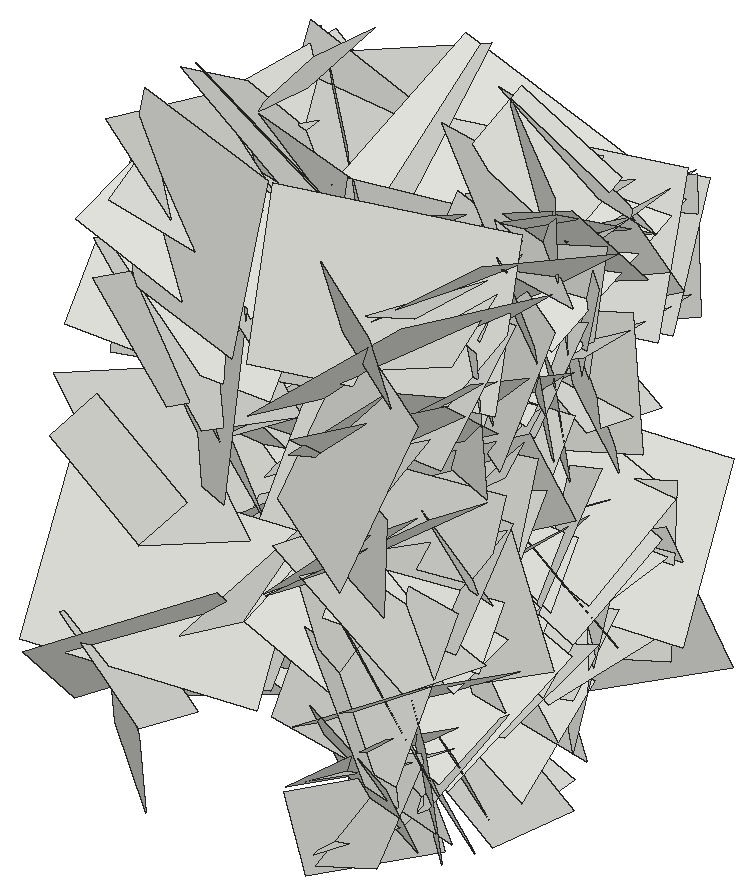
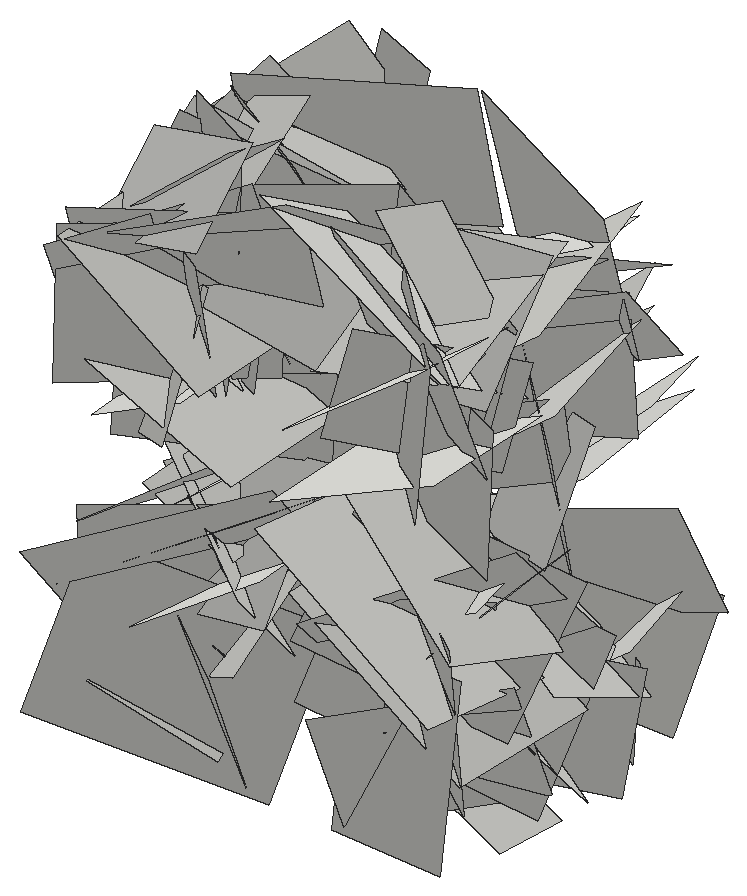
# SketchUp Ruby script. Lengths in inches.
U = 1.inch
M = Sketchup.active_model
def pt(a) = Geom::Point3d.new(a.map { |v| v * U })
def face(e, loops, mat)
  f = e.add_face(loops[0].map { |a| pt(a) })
  loops[1..].each { |l| e.add_face(l.map { |a| pt(a) }).erase! }
  f.material = f.back_material = mat if mat
  f
end
# faces: each face lists its corners as indices into pts; further lists are holes
def faces(e, pts, list, mat = nil) = list.each { |f| face(e, (f[0].is_a?(Array) ? f : [f]).map { |l| l.map { |i| pts[i] } }, mat) }
# xy, xz, yz: faces in a plane at the given z, y or x. An outline is a flat list of corners, or four numbers for a rectangle; further outlines are holes
def ring(l) = l.size == 4 ? [[l[0], l[1]], [l[2], l[1]], [l[2], l[3]], [l[0], l[3]]] : l.each_slice(2).to_a
def flat(e, list, mat, &to3) = list.each { |f| face(e, (f[0].is_a?(Array) ? f : [f]).map { |l| ring(l).map { |u, v| to3.(u, v) } }, mat) }
def xy(e, z, list, mat = nil) = flat(e, list, mat) { |x, y| [x, y, z] }
def xz(e, y, list, mat = nil) = flat(e, list, mat) { |x, z| [x, y, z] }
def yz(e, x, list, mat = nil) = flat(e, list, mat) { |y, z| [x, y, z] }
def lines(e, pts, list) = list.each { |a, b| e.add_line(pt(pts[a]), pt(pts[b])) }
# prism: a flat outline (further loops are holes) pulled along v
def prism(e, loops, v, mat = nil)
  f = face(e, loops, mat); d = Geom::Vector3d.new(v.map { |x| x * U })
  f.pushpull(f.normal.samedirection?(d) ? d.length : -d.length)
end
def box(e, o, s, mat = nil) = prism(e, [[o, [o[0] + s[0], o[1], o[2]], [o[0] + s[0], o[1] + s[1], o[2]], [o[0], o[1] + s[1], o[2]]]], [0, 0, s[2]], mat)
def at(x, y, z, deg = 0) = Geom::Transformation.translation(pt([x, y, z])) * Geom::Transformation.rotation(ORIGIN, Z_AXIS, deg.degrees)
def axes(o, x, y, z) = Geom::Transformation.new([*x, 0, *y, 0, *z, 0, *pt(o).to_a, 1])
def part(name) = M.definitions.add(name)
# library, detail: a bought-in or finely detailed component or shape, given as its bounding box
def library(name, o, s) = part(name).tap { |d| box(d.entities, o, s) }
def detail(e, o, s) = box(e.add_group.entities, o, s)
def put(e, d, t, mat = nil) = e.add_instance(d, t).tap { |i| i.material = mat if mat }
def group(e, t, mat = nil) = e.add_group.tap { |g| g.transformation = t; g.material = mat if mat }.entities
root = M.entities
c1 = part("Component\#6")
p = [[0.01,0,0],[0,3.24,4.54],[4.32,3.24,4.54],[4.33,0,0]]
faces(c1.entities,p,[[0,1,2,3]])
put(root,c1,axes([14.53,182.77,28.15],[-0.11013,-1.0722,-0.31704],[-0.03816,-0.31503,1.07721],[1.18456,-0.10983,0.00522]))
put(root,c1,axes([14.53,176.05,33.17],[0.01986,0.50916,-0.88553],[-0.06176,-0.8837,-0.50934],[1.08099,-0.05984,-0.01283]))
put(root,c1,axes([18.5,182.27,37.76],[0.22679,0.05489,-0.89691],[0.06736,-0.9206,-0.04118],[-0.95012,-0.05216,-0.217]))
put(root,c1,axes([14.53,174.9,23.69],[-0.06803,0.90477,0.33383],[0.16872,0.33992,-0.89067],[1.00823,0.00417,0.17157]))
put(root,c1,axes([18.5,173.11,21.9],[0.05319,-0.68826,0.19248],[0.04456,0.19546,0.68797],[-0.75624,-0.03689,0.05408]))
put(root,c1,axes([18.5,178.15,33.23],[-0.08938,-0.00525,-0.60269],[0.06829,-0.60515,-0.00374],[-0.63521,-0.06432,0.0844]))
put(root,c1,axes([18.5,176.44,21.6],[0.04345,0.60879,-0.00304],[-0.10651,0.00376,-0.60183],[-0.63647,0.04093,0.10051]))
put(root,c1,axes([14.53,183.67,38.38],[0.04708,0.10578,-1.15378],[-0.2342,-1.13267,-0.11235],[1.2056,-0.22416,0.02323]))
put(root,c1,axes([14.53,173.31,35.98],[-0.01252,1.07454,-0.37217],[-0.12805,-0.37127,-1.06811],[1.19858,-0.02844,-0.11799]))
put(root,c1,axes([14.53,174.78,20.26],[0.10048,-0.39109,0.79293],[0.10042,0.79738,0.38196],[0.93179,-0.04376,-0.12667]))
put(root,c1,axes([18.5,180.68,27.18],[0.06604,-0.60003,0.10008],[-0.10227,0.08959,0.59716],[-0.63666,-0.07663,-0.08554]))
put(root,c1,axes([18.5,170.73,19.61],[0.06378,-0.15247,0.68566],[0.07422,0.68605,0.14641],[-0.74085,0.05561,0.0737]))
put(root,c1,axes([14.53,178.01,21.81],[0.00864,0.40014,0.99077],[-0.02339,0.99065,-0.39991],[1.13239,0.01741,-0.01582]))
put(root,c1,axes([18.5,178.13,40.15],[0.04908,0.64392,0.19174],[0.08573,0.18545,-0.64234],[-0.70699,0.06719,-0.06458]))
put(root,c1,axes([14.53,171.95,33.74],[-0.07102,0.70639,0.8167],[0.11892,0.8184,-0.69866],[1.13841,-0.04142,0.12393]))
put(root,c1,axes([18.5,176.07,37.03],[0.15674,-0.62528,-0.09698],[-0.10666,-0.12156,0.63036],[-0.66219,-0.12843,-0.12449]))
put(root,c1,axes([18.5,180.42,25.12],[0.17902,-0.88337,-0.09354],[0.21931,-0.05348,0.8786],[-0.91571,-0.1855,0.19214]))
put(root,c1,axes([14.53,172.46,21.25],[0.14489,-0.73421,0.72244],[-0.08794,0.71856,0.74596],[1.0883,0.15581,-0.0359]))
put(root,c1,axes([14.53,171.47,32.36],[0.16942,0.96147,-0.31887],[-0.08969,-0.30901,-0.97416],[1.06999,-0.17814,-0.03117]))
put(root,c1,axes([14.53,179.35,38.14],[0.07028,1.07405,0.02302],[-0.04111,0.02544,-1.07534],[1.13802,-0.06541,-0.04027]))
put(root,c1,axes([18.5,181.39,28.46],[0.11732,-0.15238,-0.58962],[-0.01785,-0.59981,0.15186],[-0.64528,-0.01111,-0.1114]))
put(root,c1,axes([18.5,173.74,31.89],[0.15856,-0.67469,0.29232],[0.1064,0.31425,0.67394],[-0.77211,-0.09525,0.1529]))
put(root,c1,axes([14.53,173.84,39.64],[-0.13369,1.27699,-0.41872],[-0.11509,-0.42887,-1.27523],[1.41986,0.08547,-0.14279]))
put(root,c1,axes([18.5,172.58,29],[0.14706,-0.68518,0.03236],[0.10474,0.05263,0.69082],[-0.71951,-0.13238,0.10718]))
put(root,c1,axes([14.53,180.75,35.09],[-0.01445,0.08276,-1.11066],[0.1396,-1.10283,-0.0838],[1.17228,0.13235,-0.00371]))
put(root,c1,axes([14.53,182.25,27.43],[-0.1955,0.46825,-1.21407],[0.10064,-1.21809,-0.48422],[1.37564,0.15566,-0.13711]))
put(root,c1,axes([14.53,175.96,26.52],[0.03553,0.82214,0.9074],[-0.07429,0.90754,-0.81968],[1.2958,0.02948,-0.07187]))
put(root,c1,axes([14.53,172.47,36.95],[0.1233,0.89549,0.4145],[0.21728,0.38634,-0.89217],[1.02316,-0.18996,0.13951]))
put(root,c1,axes([14.53,183.25,38.77],[-0.07927,-0.40868,-1.12281],[0.1988,-1.11508,0.39337],[1.25087,0.15132,-0.13368]))
put(root,c1,axes([14.53,179.04,23.77],[0.11323,-0.75693,-0.7774],[0.09292,-0.77258,0.76428],[1.14637,0.13739,0.01483]))
put(root,c1,axes([14.53,182.77,28.7],[-0.0358,-0.11408,-1.31406],[-0.04325,-1.31377,0.1151],[1.39747,-0.04358,-0.0301]))
put(root,c1,axes([14.53,180.07,24.39],[-0.06666,-0.76105,0.92501],[0.21989,0.90537,0.75899],[1.25053,-0.19976,-0.08415]))
put(root,c1,axes([14.53,177.97,39.67],[-0.02985,0.75948,-0.84861],[0.27983,-0.8214,-0.74388],[1.17429,0.21504,0.15569]))
put(root,c1,axes([14.53,174.06,31.875],[0.08593,-0.00736,1.08266],[0.18405,1.07173,-0.00571],[1.1328,-0.17357,-0.0812]))
put(root,c1,axes([14.53,182.31,23.94],[-0.04872,-1.30982,0.04089],[0.01644,0.04037,1.31055],[1.38898,-0.04642,-0.01408]))
put(root,c1,axes([14.53,178.49,34.59],[0.00763,1.14917,-0.03145],[0.21412,-0.03223,-1.13128],[1.19962,-0.00155,0.20212]))
put(root,c1,axes([14.53,178.09,32.9],[0.18757,-0.47698,-1.21124],[-0.23196,-1.21588,0.44684],[1.36024,-0.14157,0.24323]))
put(root,c1,axes([14.53,178.68,21.25],[0.14964,-1.02559,0.91665],[-0.24358,0.89093,1.03221],[1.43757,0.25771,0.07948]))
put(root,c1,axes([14.53,169.91,24.28],[-0.0494,0.58776,1.07494],[0.25393,1.05932,-0.56884],[1.27358,-0.18841,0.15511]))
put(root,c1,axes([14.53,175.66,39.88],[-0.03914,-0.32872,-1.22009],[0.25418,-1.20026,0.31612],[1.31508,0.2222,-0.09741]))
put(root,c1,axes([14.53,177.96,25.04],[0.10915,-1.1796,-0.55067],[0.03689,-0.5497,1.18402],[1.37942,0.10803,0.01191]))
put(root,c1,axes([14.53,183.77,26.5],[0.0762,-1.33255,-0.21023],[0.04546,-0.20817,1.33413],[1.42926,0.07766,-0.03122]))
put(root,c1,axes([14.53,177.28,39.83],[0.04784,1.11638,-0.64936],[0.22797,-0.64718,-1.09769],[1.34988,0.06974,0.20839]))
put(root,c1,axes([14.53,179.625,37.91],[0.28026,0.12179,-1.29213],[0.26115,-1.29941,-0.07206],[1.35072,0.22596,0.28204]))
put(root,c1,axes([14.53,183.19,37.72],[0.19709,-1.17807,-0.70591],[0.26547,-0.67132,1.18631],[1.43137,0.28672,-0.12282]))
put(root,c1,axes([28.31,183.19,37.72],[-0.19709,-1.17807,-0.70591],[-0.26547,-0.67132,1.18631],[-1.43137,0.28672,-0.12282]))
put(root,c1,axes([28.31,179.625,37.91],[-0.28026,0.12179,-1.29213],[-0.26115,-1.29941,-0.07206],[-1.35072,0.22596,0.28204]))
put(root,c1,axes([28.31,177.28,39.83],[-0.04784,1.11638,-0.64936],[-0.22797,-0.64718,-1.09769],[-1.34988,0.06974,0.20839]))
put(root,c1,axes([28.31,183.77,26.5],[-0.0762,-1.33255,-0.21023],[-0.04546,-0.20817,1.33413],[-1.42926,0.07766,-0.03122]))
put(root,c1,axes([28.31,177.96,25.04],[-0.10915,-1.1796,-0.55067],[-0.03689,-0.5497,1.18402],[-1.37942,0.10803,0.01191]))
put(root,c1,axes([28.31,175.66,39.88],[0.03914,-0.32872,-1.22009],[-0.25418,-1.20026,0.31612],[-1.31508,0.2222,-0.09741]))
put(root,c1,axes([28.31,169.91,24.28],[0.0494,0.58776,1.07494],[-0.25393,1.05932,-0.56884],[-1.27358,-0.18841,0.15511]))
put(root,c1,axes([28.31,178.68,21.25],[-0.14964,-1.02559,0.91665],[0.24358,0.89093,1.03221],[-1.43757,0.25771,0.07948]))
put(root,c1,axes([28.31,178.09,32.9],[-0.18757,-0.47698,-1.21124],[0.23196,-1.21588,0.44684],[-1.36024,-0.14157,0.24323]))
put(root,c1,axes([28.31,178.49,34.59],[-0.00763,1.14917,-0.03145],[-0.21412,-0.03223,-1.13128],[-1.19962,-0.00155,0.20212]))
put(root,c1,axes([28.31,182.31,23.94],[0.04872,-1.30982,0.04089],[-0.01644,0.04037,1.31055],[-1.38898,-0.04642,-0.01408]))
put(root,c1,axes([28.31,174.06,31.875],[-0.08593,-0.00736,1.08266],[-0.18405,1.07173,-0.00571],[-1.1328,-0.17357,-0.0812]))
put(root,c1,axes([28.31,177.97,39.67],[0.02985,0.75948,-0.84861],[-0.27983,-0.8214,-0.74388],[-1.17429,0.21504,0.15569]))
put(root,c1,axes([28.31,180.07,24.39],[0.06666,-0.76105,0.92501],[-0.21989,0.90537,0.75899],[-1.25053,-0.19976,-0.08415]))
put(root,c1,axes([28.31,182.77,28.7],[0.0358,-0.11408,-1.31406],[0.04325,-1.31377,0.1151],[-1.39747,-0.04358,-0.0301]))
put(root,c1,axes([28.31,179.04,23.77],[-0.11323,-0.75693,-0.7774],[-0.09292,-0.77258,0.76428],[-1.14637,0.13739,0.01483]))
put(root,c1,axes([28.31,183.25,38.77],[0.07927,-0.40868,-1.12281],[-0.1988,-1.11508,0.39337],[-1.25087,0.15132,-0.13368]))
put(root,c1,axes([28.31,172.47,36.95],[-0.1233,0.89549,0.4145],[-0.21728,0.38634,-0.89217],[-1.02316,-0.18996,0.13951]))
put(root,c1,axes([28.31,175.96,26.52],[-0.03553,0.82214,0.9074],[0.07429,0.90754,-0.81968],[-1.2958,0.02948,-0.07187]))
put(root,c1,axes([28.31,182.25,27.43],[0.1955,0.46825,-1.21407],[-0.10064,-1.21809,-0.48422],[-1.37564,0.15566,-0.13711]))
put(root,c1,axes([28.31,180.75,35.09],[0.01445,0.08276,-1.11066],[-0.1396,-1.10283,-0.0838],[-1.17228,0.13235,-0.00371]))
put(root,c1,axes([24.34,172.58,29],[-0.14706,-0.68518,0.03236],[-0.10474,0.05263,0.69082],[0.71951,-0.13238,0.10718]))
put(root,c1,axes([28.31,173.84,39.64],[0.13369,1.27699,-0.41872],[0.11509,-0.42887,-1.27523],[-1.41986,0.08547,-0.14279]))
put(root,c1,axes([24.34,173.74,31.89],[-0.15856,-0.67469,0.29232],[-0.1064,0.31425,0.67394],[0.77211,-0.09525,0.1529]))
put(root,c1,axes([24.34,181.39,28.46],[-0.11732,-0.15238,-0.58962],[0.01785,-0.59981,0.15186],[0.64528,-0.01111,-0.1114]))
put(root,c1,axes([28.31,179.35,38.14],[-0.07028,1.07405,0.02302],[0.04111,0.02544,-1.07534],[-1.13802,-0.06541,-0.04027]))
put(root,c1,axes([28.31,171.47,32.36],[-0.16942,0.96147,-0.31887],[0.08969,-0.30901,-0.97416],[-1.06999,-0.17814,-0.03117]))
put(root,c1,axes([28.31,172.46,21.25],[-0.14489,-0.73421,0.72244],[0.08794,0.71856,0.74596],[-1.0883,0.15581,-0.0359]))
put(root,c1,axes([24.34,180.42,25.12],[-0.17902,-0.88337,-0.09354],[-0.21931,-0.05348,0.8786],[0.91571,-0.1855,0.19214]))
put(root,c1,axes([24.34,176.07,37.03],[-0.15674,-0.62528,-0.09698],[0.10666,-0.12156,0.63036],[0.66219,-0.12843,-0.12449]))
put(root,c1,axes([28.31,171.95,33.74],[0.07102,0.70639,0.8167],[-0.11892,0.8184,-0.69866],[-1.13841,-0.04142,0.12393]))
put(root,c1,axes([24.34,178.13,40.15],[-0.04908,0.64392,0.19174],[-0.08573,0.18545,-0.64234],[0.70699,0.06719,-0.06458]))
put(root,c1,axes([28.31,178.01,21.81],[-0.00864,0.40014,0.99077],[0.02339,0.99065,-0.39991],[-1.13239,0.01741,-0.01582]))
put(root,c1,axes([24.34,170.73,19.61],[-0.06378,-0.15247,0.68566],[-0.07422,0.68605,0.14641],[0.74085,0.05561,0.0737]))
put(root,c1,axes([24.34,180.68,27.18],[-0.06604,-0.60003,0.10008],[0.10227,0.08959,0.59716],[0.63666,-0.07663,-0.08554]))
put(root,c1,axes([28.31,174.78,20.26],[-0.10048,-0.39109,0.79293],[-0.10042,0.79738,0.38196],[-0.93179,-0.04376,-0.12667]))
put(root,c1,axes([28.31,173.31,35.98],[0.01252,1.07454,-0.37217],[0.12805,-0.37127,-1.06811],[-1.19858,-0.02844,-0.11799]))
put(root,c1,axes([28.31,183.67,38.38],[-0.04708,0.10578,-1.15378],[0.2342,-1.13267,-0.11235],[-1.2056,-0.22416,0.02323]))
put(root,c1,axes([24.34,176.44,21.6],[-0.04345,0.60879,-0.00304],[0.10651,0.00376,-0.60183],[0.63647,0.04093,0.10051]))
put(root,c1,axes([24.34,178.15,33.23],[0.08938,-0.00525,-0.60269],[-0.06829,-0.60515,-0.00374],[0.63521,-0.06432,0.0844]))
put(root,c1,axes([24.34,173.11,21.9],[-0.05319,-0.68826,0.19248],[-0.04456,0.19546,0.68797],[0.75624,-0.03689,0.05408]))
put(root,c1,axes([28.31,174.9,23.69],[0.06803,0.90477,0.33383],[-0.16872,0.33992,-0.89067],[-1.00823,0.00417,0.17157]))
put(root,c1,axes([24.34,182.27,37.76],[-0.22679,0.05489,-0.89691],[-0.06736,-0.9206,-0.04118],[0.95012,-0.05216,-0.217]))
put(root,c1,axes([28.31,176.05,33.17],[-0.01986,0.50916,-0.88553],[0.06176,-0.8837,-0.50934],[-1.08099,-0.05984,-0.01283]))
put(root,c1,axes([28.31,182.77,28.15],[0.11013,-1.0722,-0.31704],[0.03816,-0.31503,1.07721],[-1.18456,-0.10983,0.00522]))
put(root,c1,axes([28.31,185.38,28.27],[0.28552,-0.8956,-0.93898],[0.07116,-0.9481,0.92355],[-1.37362,-0.23528,-0.14733]))
put(root,c1,axes([24.34,175.43,34.87],[-0.0411,0.62613,0.35799],[-0.03637,0.3565,-0.62724],[0.76365,0.05068,-0.01061]))
put(root,c1,axes([24.34,173.67,32.24],[-0.05341,-0.65994,-0.37026],[-0.06447,-0.36634,0.66124],[0.79951,-0.07362,0.02859]))
put(root,c1,axes([28.31,174.01,26.46],[0.07872,-0.97306,0.24072],[-0.0738,0.23579,0.97461],[-1.05998,-0.08868,-0.04998]))
put(root,c1,axes([28.31,170.16,39.2],[0.24703,1.2789,-0.21613],[0.13589,-0.24123,-1.28918],[-1.36812,0.20696,-0.16707]))
put(root,c1,axes([24.34,173.15,22.23],[0.01199,-0.5915,0.12784],[0.10227,0.12799,0.58366],[0.63327,-0.00947,-0.09668]))
put(root,c1,axes([28.31,167.34,31.77],[0.2501,0.51374,1.1242],[0.05799,1.13903,-0.532],[-1.3089,0.14863,0.19123]))
put(root,c1,axes([24.34,174.375,32.02],[-0.18574,0.64681,-0.5499],[-0.00393,-0.56207,-0.65994],[0.8999,0.13105,-0.11638]))
put(root,c1,axes([24.34,171.42,39.46],[0.01769,0.21401,-0.61924],[0.03571,-0.6189,-0.21298],[0.69357,0.02641,0.02676]))
put(root,c1,axes([24.34,180.11,41],[-0.0874,0.13713,-0.78202],[-0.02965,-0.78624,-0.13492],[0.84107,-0.01347,-0.08602]))
put(root,c1,axes([28.31,182.1,27.04],[0.18817,-1.1788,-0.21223],[0.10509,-0.19936,1.19019],[-1.26526,-0.19187,0.06729]))
put(root,c1,axes([28.31,177.13,31.79],[0.078,-0.30439,1.03044],[0.07955,1.03178,0.29943],[-1.13614,0.05135,0.09171]))
put(root,c1,axes([28.31,172.13,35.78],[-0.07615,0.65901,-0.5201],[-0.04859,-0.52431,-0.658],[-0.88857,-0.02781,0.08055]))
put(root,c1,axes([28.31,172.625,27.43],[0.01975,0.58315,0.74345],[-0.01761,0.74368,-0.58292],[-1.00141,-0.00157,0.02491]))
put(root,c1,axes([28.31,173.5,20.5],[0.29119,-0.77592,0.90535],[-0.00734,0.92801,0.79744],[-1.26387,-0.18415,0.20396]))
put(root,c1,axes([28.31,181.8125,37.17],[0.0246,-0.63961,0.56311],[-0.17949,0.54862,0.63013],[-0.88529,-0.129,-0.11211]))
put(root,c1,axes([24.34,177.7,39.03],[-0.08239,-0.33737,-0.64844],[0.10668,-0.65083,0.32654],[0.76743,0.05425,-0.11501]))
put(root,c1,axes([28.31,176.41,32.2],[-0.11408,-0.0942,-0.79779],[-0.0272,-0.8041,0.09841],[-0.85109,0.03832,0.10379]))
put(root,c1,axes([28.31,171.36,22.89],[-0.02535,0.88672,0.32576],[0.06435,0.32663,-0.88464],[-0.99927,-0.00146,-0.06523]))
put(root,c1,axes([28.31,178.05,19.9375],[0.14578,-1.0409,0.22357],[0.02192,0.228,1.04879],[-1.1283,-0.13006,0.04926]))
put(root,c1,axes([28.31,180.04,24.28],[-0.15161,0.71603,-0.23582],[-0.04269,-0.24694,-0.72538],[-0.79796,-0.12284,0.08362]))
put(root,c1,axes([24.34,173.29,20.87],[0.09428,-0.62013,-0.08152],[0.03551,-0.0775,0.6261],[0.66205,0.09247,-0.02197]))
put(root,c1,axes([24.34,173.36,27.66],[-0.12062,0.63946,0.63128],[-0.06443,0.62939,-0.6485],[0.9503,0.12384,0.03616]))
put(root,c1,axes([28.31,175.14,30.45],[0.22771,0.17317,-1.07869],[-0.0194,-1.09862,-0.18001],[-1.15789,0.05246,-0.20912]))
put(root,c1,axes([28.31,184.3,37.98],[0.01849,-0.42221,-1.00939],[0.24573,-0.98518,0.41609],[-1.13346,-0.22047,0.07374]))
put(root,c1,axes([24.34,172.01,32.68],[0.01531,-0.04852,-0.71126],[0.05574,-0.70939,0.04946],[0.75363,0.05345,0.01079]))
put(root,c1,axes([28.31,172,20.82],[0.19013,-0.4174,1.11707],[0.18593,1.12659,0.39279],[-1.25031,0.10406,0.22828]))
put(root,c1,axes([28.31,178.01,36.42],[-0.04909,-0.68925,0.58112],[0.09024,0.57594,0.68989],[-0.95135,0.0902,0.03545]))
put(root,c1,axes([28.31,174.95,31.63],[-0.12097,-0.07785,-0.70642],[-0.09105,-0.70871,0.09198],[-0.74781,0.09888,0.10307]))
put(root,c1,axes([24.34,171.52,27.71],[-0.03995,0.48298,0.66079],[-0.01207,0.66111,-0.48387],[0.8675,0.03144,0.0237]))
put(root,c1,axes([28.31,174.16,29.86],[-0.19319,0.59277,-0.26834],[-0.07097,-0.29428,-0.60458],[-0.68606,-0.13648,0.1381]))
put(root,c1,axes([28.31,171.18,26.98],[0.09963,0.88743,-0.23237],[-0.05305,-0.22828,-0.89204],[-0.97094,0.10354,0.02489]))
put(root,c1,axes([28.31,169.05,21.98],[-0.04882,0.58162,0.59704],[0.02934,0.59868,-0.58109],[-0.88303,-0.01226,-0.05232]))
put(root,c1,axes([28.31,176.26,32.94],[-0.03084,0.60524,0.59943],[0.03406,0.60013,-0.60439],[-0.90231,0.00196,-0.0433]))
put(root,c1,axes([28.31,174.875,32.24],[-0.12053,0.70886,0.38052],[0.08644,0.39248,-0.70676],[-0.84842,-0.06072,-0.12606]))
put(root,c1,axes([28.31,177.89,30.77],[-0.05678,-0.11721,0.8526],[0.09083,0.84928,0.12214],[-0.90772,0.09231,-0.04111]))
put(root,c1,axes([28.31,177.99,23.55],[-0.04107,0.5427,0.4395],[-0.20397,0.41484,-0.52921],[-0.71159,-0.15024,0.12632]))
put(root,c1,axes([28.31,174.67,32.54],[0.17055,0.3665,0.95024],[0.03456,0.95968,-0.37566],[-1.07902,0.08867,0.13816]))
put(root,c1,axes([28.31,176.52,27.27],[-0.06139,-0.83333,-0.30669],[0.14477,-0.31205,0.82208],[-0.93005,0.00643,0.1482]))
put(root,c1,axes([24.34,180.66,33.34],[-0.08177,-0.45253,0.73357],[0.03972,0.73405,0.45677],[0.91278,-0.07248,0.04584]))
put(root,c1,axes([24.34,181.67,36.78],[-0.05967,0.56874,-0.94691],[-0.29528,-0.9248,-0.5389],[1.13301,-0.21107,-0.19031]))
put(root,c1,axes([24.34,170.91,25.11],[0.00896,0.33986,-0.6335],[0.15678,-0.62081,-0.33108],[0.74574,0.12644,0.07722]))
put(root,c1,axes([28.31,182.09,31.375],[-0.0562,-0.72005,0.10613],[-0.07977,0.11126,0.71729],[-0.76737,0.04117,-0.08234]))
